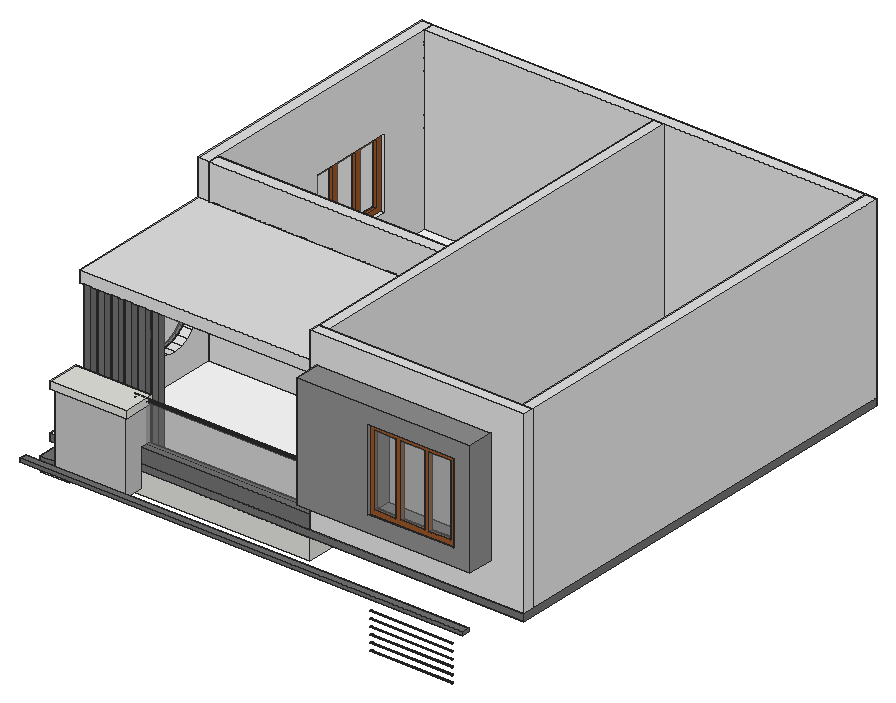
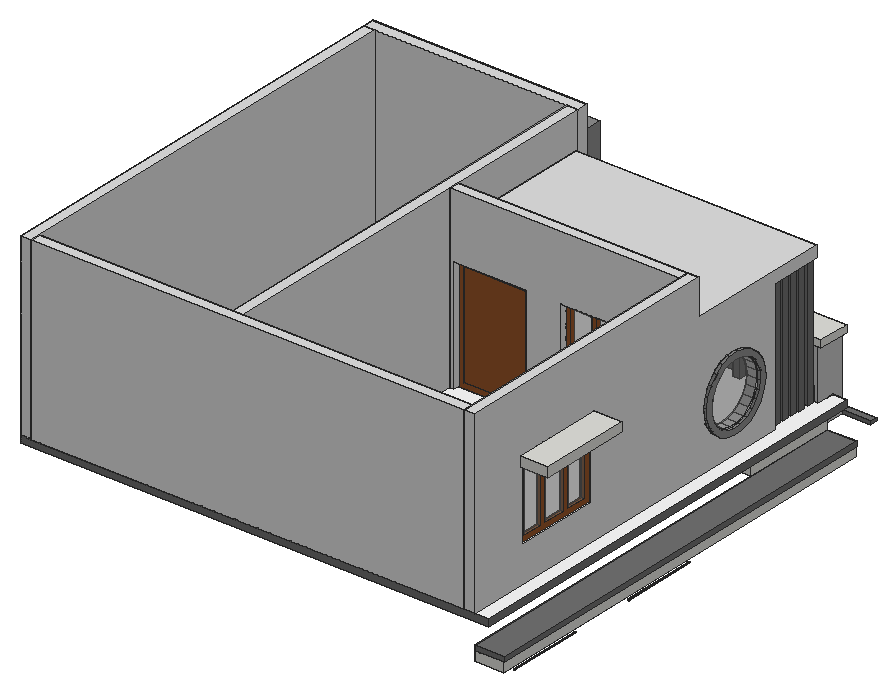
# SketchUp Ruby script. Lengths in inches.
U = 1.inch
M = Sketchup.active_model
def pt(a) = Geom::Point3d.new(a.map { |v| v * U })
def face(e, loops, mat)
  f = e.add_face(loops[0].map { |a| pt(a) })
  loops[1..].each { |l| e.add_face(l.map { |a| pt(a) }).erase! }
  f.material = f.back_material = mat if mat
  f
end
# faces: each face lists its corners as indices into pts; further lists are holes
def faces(e, pts, list, mat = nil) = list.each { |f| face(e, (f[0].is_a?(Array) ? f : [f]).map { |l| l.map { |i| pts[i] } }, mat) }
# xy, xz, yz: faces in a plane at the given z, y or x. An outline is a flat list of corners, or four numbers for a rectangle; further outlines are holes
def ring(l) = l.size == 4 ? [[l[0], l[1]], [l[2], l[1]], [l[2], l[3]], [l[0], l[3]]] : l.each_slice(2).to_a
def flat(e, list, mat, &to3) = list.each { |f| face(e, (f[0].is_a?(Array) ? f : [f]).map { |l| ring(l).map { |u, v| to3.(u, v) } }, mat) }
def xy(e, z, list, mat = nil) = flat(e, list, mat) { |x, y| [x, y, z] }
def xz(e, y, list, mat = nil) = flat(e, list, mat) { |x, z| [x, y, z] }
def yz(e, x, list, mat = nil) = flat(e, list, mat) { |y, z| [x, y, z] }
def lines(e, pts, list) = list.each { |a, b| e.add_line(pt(pts[a]), pt(pts[b])) }
# prism: a flat outline (further loops are holes) pulled along v
def prism(e, loops, v, mat = nil)
  f = face(e, loops, mat); d = Geom::Vector3d.new(v.map { |x| x * U })
  f.pushpull(f.normal.samedirection?(d) ? d.length : -d.length)
end
def box(e, o, s, mat = nil) = prism(e, [[o, [o[0] + s[0], o[1], o[2]], [o[0] + s[0], o[1] + s[1], o[2]], [o[0], o[1] + s[1], o[2]]]], [0, 0, s[2]], mat)
def at(x, y, z, deg = 0) = Geom::Transformation.translation(pt([x, y, z])) * Geom::Transformation.rotation(ORIGIN, Z_AXIS, deg.degrees)
def axes(o, x, y, z) = Geom::Transformation.new([*x, 0, *y, 0, *z, 0, *pt(o).to_a, 1])
def part(name) = M.definitions.add(name)
# library, detail: a bought-in or finely detailed component or shape, given as its bounding box
def library(name, o, s) = part(name).tap { |d| box(d.entities, o, s) }
def detail(e, o, s) = box(e.add_group.entities, o, s)
def put(e, d, t, mat = nil) = e.add_instance(d, t).tap { |i| i.material = mat if mat }
def group(e, t, mat = nil) = e.add_group.tap { |g| g.transformation = t; g.material = mat if mat }.entities
root = M.entities
M.materials.add("[Color M00]").color = [255, 255, 255]
M.materials.add("[Color M01]").color = [226, 226, 226]
M.materials.add("[Color M02]").color = [198, 198, 198]
M.materials.add("[Color M04]").color = [142, 142, 142]
M.materials.add("[Color M05]").color = [114, 114, 114]
M.materials.add("[Metal Silver]").color = [234, 233, 238]
M.materials.add("[Translucent Glass Gray]").color = [128, 128, 128]
M.materials["[Translucent Glass Gray]"].alpha = 0.5
M.materials.add("[Wood Cherry Original]").color = [152, 86, 42]
c1 = part("Group\#25")
prism(c1.entities,[[[0.28,64,0.08],[0.16,64,0.16],[0.08,64,0.28],[0.02,64,0.42],[0,64,0.5625],[0.02,64,0.71],[0.08,64,0.84],[0.16,64,0.96],[0.28,64,1.05],[0.42,64,1.11],[0.5625,64,1.125],[0.71,64,1.11],[0.84,64,1.05],[0.96,64,0.96],[1.05,64,0.84],[1.11,64,0.71],[1.125,64,0.5625],[1.11,64,0.42],[1.05,64,0.28],[0.96,64,0.16],[0.84,64,0.08],[0.71,64,0.02],[0.5625,64,0],[0.42,64,0.02]]],[0,-64,0])
c2 = part("Group\#30")
prism(c2.entities,[[[0.15,64,0.15],[0.07,64,0.25],[0.02,64,0.37],[0,64,0.5],[0.02,64,0.63],[0.07,64,0.75],[0.15,64,0.85],[0.25,64,0.93],[0.37,64,0.98],[0.5,64,1],[0.63,64,0.98],[0.75,64,0.93],[0.85,64,0.85],[0.93,64,0.75],[0.98,64,0.63],[1,64,0.5],[0.98,64,0.37],[0.93,64,0.25],[0.85,64,0.15],[0.75,64,0.07],[0.63,64,0.02],[0.5,64,0],[0.37,64,0.02],[0.25,64,0.07]]],[0,-64,0])
c3 = part("Group\#18")
prism(c3.entities,[[[0,1.11,0.71],[0,1.125,0.5625],[0,1.11,0.42],[0,1.05,0.28],[0,0.96,0.16],[0,0.84,0.08],[0,0.71,0.02],[0,0.5625,0],[0,0.42,0.02],[0,0.28,0.08],[0,0.16,0.16],[0,0.08,0.28],[0,0.02,0.42],[0,0,0.5625],[0,0.02,0.71],[0,0.08,0.84],[0,0.16,0.96],[0,0.28,1.05],[0,0.42,1.11],[0,0.5625,1.125],[0,0.71,1.11],[0,0.84,1.05],[0,0.96,0.96],[0,1.05,0.84]]],[64,0,0])
c4 = part("Group\#73")
box(c4.entities,[0,0,0],[6,4.96,110])
g1 = group(root,at(352.33,147.5,84.5))
prism(g1,[[[64,0.11,0.64],[64,0.05,0.5625],[64,0.01,0.47],[64,0,0.375],[64,0.01,0.28],[64,0.05,0.1875],[64,0.11,0.11],[64,0.1875,0.05],[64,0.28,0.01],[64,0.375,0],[64,0.47,0.01],[64,0.5625,0.05],[64,0.64,0.11],[64,0.7,0.1875],[64,0.74,0.28],[64,0.75,0.375],[64,0.74,0.47],[64,0.7,0.5625],[64,0.64,0.64],[64,0.5625,0.7],[64,0.47,0.74],[64,0.375,0.75],[64,0.28,0.74],[64,0.1875,0.7]]],[-69,0,0])
put(root,c1,at(87.27,300.375,86.45))
put(root,c2,at(87.33,420.375,86.78))
put(root,c3,at(137.33,242.3125,89.07))
g2 = group(root,at(352.33,147.5,90.5))
prism(g2,[[[64,0.11,0.64],[64,0.05,0.5625],[64,0.01,0.47],[64,0,0.375],[64,0.01,0.28],[64,0.05,0.1875],[64,0.11,0.11],[64,0.1875,0.05],[64,0.28,0.01],[64,0.375,0],[64,0.47,0.01],[64,0.5625,0.05],[64,0.64,0.11],[64,0.7,0.1875],[64,0.74,0.28],[64,0.75,0.375],[64,0.74,0.47],[64,0.7,0.5625],[64,0.64,0.64],[64,0.5625,0.7],[64,0.47,0.74],[64,0.375,0.75],[64,0.28,0.74],[64,0.1875,0.7]]],[-69,0,0])
put(root,c1,at(87.27,300.375,92.45))
put(root,c2,at(87.33,420.375,92.78))
put(root,c3,at(137.33,242.3125,95.07))
g3 = group(root,at(352.33,147.5,96.5))
prism(g3,[[[64,0.11,0.64],[64,0.05,0.5625],[64,0.01,0.47],[64,0,0.375],[64,0.01,0.28],[64,0.05,0.1875],[64,0.11,0.11],[64,0.1875,0.05],[64,0.28,0.01],[64,0.375,0],[64,0.47,0.01],[64,0.5625,0.05],[64,0.64,0.11],[64,0.7,0.1875],[64,0.74,0.28],[64,0.75,0.375],[64,0.74,0.47],[64,0.7,0.5625],[64,0.64,0.64],[64,0.5625,0.7],[64,0.47,0.74],[64,0.375,0.75],[64,0.28,0.74],[64,0.1875,0.7]]],[-69,0,0])
put(root,c1,at(87.27,300.375,98.45))
put(root,c2,at(87.33,420.375,98.78))
put(root,c3,at(137.33,242.3125,101.07))
g4 = group(root,at(352.33,147.5,102.5))
prism(g4,[[[64,0.11,0.64],[64,0.05,0.5625],[64,0.01,0.47],[64,0,0.375],[64,0.01,0.28],[64,0.05,0.1875],[64,0.11,0.11],[64,0.1875,0.05],[64,0.28,0.01],[64,0.375,0],[64,0.47,0.01],[64,0.5625,0.05],[64,0.64,0.11],[64,0.7,0.1875],[64,0.74,0.28],[64,0.75,0.375],[64,0.74,0.47],[64,0.7,0.5625],[64,0.64,0.64],[64,0.5625,0.7],[64,0.47,0.74],[64,0.375,0.75],[64,0.28,0.74],[64,0.1875,0.7]]],[-69,0,0])
put(root,c1,at(87.27,300.375,104.45))
put(root,c2,at(87.33,420.375,104.78))
put(root,c3,at(137.33,242.3125,107.07))
g5 = group(root,at(352.33,147.5,108.5))
prism(g5,[[[64,0.11,0.64],[64,0.05,0.5625],[64,0.01,0.47],[64,0,0.375],[64,0.01,0.28],[64,0.05,0.1875],[64,0.11,0.11],[64,0.1875,0.05],[64,0.28,0.01],[64,0.375,0],[64,0.47,0.01],[64,0.5625,0.05],[64,0.64,0.11],[64,0.7,0.1875],[64,0.74,0.28],[64,0.75,0.375],[64,0.74,0.47],[64,0.7,0.5625],[64,0.64,0.64],[64,0.5625,0.7],[64,0.47,0.74],[64,0.375,0.75],[64,0.28,0.74],[64,0.1875,0.7]]],[-69,0,0])
g6 = group(root,at(61.33,239.375,114))
box(g6,[0,-80,0],[24,369.8125,8])
g7 = group(root,at(352.33,147.5,114.5))
prism(g7,[[[64,0.11,0.64],[64,0.05,0.5625],[64,0.01,0.47],[64,0,0.375],[64,0.01,0.28],[64,0.05,0.1875],[64,0.11,0.11],[64,0.1875,0.05],[64,0.28,0.01],[64,0.375,0],[64,0.47,0.01],[64,0.5625,0.05],[64,0.64,0.11],[64,0.7,0.1875],[64,0.74,0.28],[64,0.75,0.375],[64,0.74,0.47],[64,0.7,0.5625],[64,0.64,0.64],[64,0.5625,0.7],[64,0.47,0.74],[64,0.375,0.75],[64,0.28,0.74],[64,0.1875,0.7]]],[-69,0,0])
g8 = group(root,at(60.33,239.375,122),"[Color M05]")
box(g8,[0,-80,0],[25,369.8125,4])
g9 = group(root,at(61.33,167.375,126))
box(g9,[24,-8,0],[202,80,18])
g10 = group(root,at(61.33,137.375,131),"[Color M05]")
box(g10,[0,0,0],[372,6,3])
g11 = group(root,at(85.33,143.375,131),"[Color M02]")
xy(g11,0,[[0,0,60,16]])
xy(g11,19,[[0,16,4,25]])
xy(g11,31,[[4,16,60,25]])
xy(g11,61,[[0,0,60,25]])
xz(g11,0,[[0,0,60,61]])
xz(g11,16,[[0,0,0,19,4,19,4,31,60,31,60,0]])
xz(g11,25,[[0,19,0,61,60,61,60,31,4,31,4,19]])
yz(g11,0,[[0,0,0,61,25,61,25,19,16,19,16,0]])
yz(g11,4,[[16,19,25,31]])
yz(g11,60,[[0,0,16,0,16,31,25,31,25,61,0,61]])
g12 = group(root,at(85.33,239.375,144),"[Color M05]")
xy(g12,0,[[-12,-86,-12,289.8125,382,289.8125,382,-80,0,-80,0,-86]])
xy(g12,6,[[-12,-86,0,-86,0,-80,382,-80,382,289.8125,-12,289.8125]],"[Color M00]")
xz(g12,-86,[[-12,0,0,6]])
xz(g12,-80,[[0,0,382,6]])
xz(g12,289.8125,[[-12,0,382,6]])
yz(g12,-12,[[-86,0,289.8125,6]])
yz(g12,0,[[-86,0,-80,6]])
yz(g12,382,[[-80,0,289.8125,6]])
g13 = group(root,at(287.33,159.375,150),"[Color M01]")
box(g13,[0,0,0],[180,9,150])
g14 = group(root,at(287.33,168.375,150),"[Color M01]")
box(g14,[0,0,0],[9,351.8125,150])
g15 = group(root,at(458.33,168.375,150),"[Color M01]")
box(g15,[0,0,0],[9,360.8125,150])
g16 = group(root,at(76.33,294.375,150),"[Color M01]")
prism(g16,[[[211,9,0],[207,9,0],[207,9,96],[147,9,96],[147,9,0],[18,9,0],[18,9,150],[211,9,150]],[[117,9,96],[45,9,96],[45,9,30],[117,9,30]]],[0,-9,0])
g17 = group(root,at(85.33,255.375,150),"[Color M01]")
xy(g17,0,[[0,-41,9,273.8125]])
xy(g17,30,[[0,152,9,224]])
xy(g17,90,[[0,152,9,224]])
xy(g17,110,[[0,-85,0,-41,9,-41,9,39,202,39,202,-85]])
xy(g17,120,[[0,-85,202,39]])
xy(g17,150,[[0,39,9,273.8125]])
xz(g17,-85,[[0,110,202,120]])
xz(g17,-41,[[0,0,9,110]])
xz(g17,39,[[9,110,202,120],[0,120,9,150]])
xz(g17,152,[[0,30,9,90]])
xz(g17,224,[[0,30,9,90]])
xz(g17,273.8125,[[0,0,9,150]])
yz(g17,-3,[[[4.67,17.04,-3.4,17.67,-11.03,20.36,-17.71,24.93,-22.97,31.08,-26.47,38.38,-27.96,46.33,-27.33,54.4,-24.64,62.03,-20.07,68.71,-13.92,73.97,-6.62,77.47,1.33,78.96,9.4,78.33,17.03,75.64,23.71,71.07,28.97,64.92,32.47,57.62,33.96,49.67,33.33,41.6,30.64,33.97,26.07,27.29,19.92,22.03,12.62,18.53],[4.4,22.04,11.07,23.28,17.19,26.22,22.35,30.63,26.18,36.23,28.44,42.63,28.96,49.4,27.72,56.07,24.78,62.19,20.37,67.35,14.77,71.18,8.37,73.44,1.6,73.96,-5.07,72.72,-11.19,69.78,-16.35,65.37,-20.18,59.77,-22.44,53.37,-22.96,46.6,-21.72,39.93,-18.78,33.81,-14.37,28.65,-8.77,24.82,-2.37,22.56]]],"[Color M04]")
yz(g17,0,[[[-41,0,-41,110,-85,110,-85,120,39,120,39,150,273.8125,150,273.8125,0],[152,30,224,90],[4.67,17.04,12.62,18.53,19.92,22.03,26.07,27.29,30.64,33.97,33.33,41.6,33.96,49.67,32.47,57.62,28.97,64.92,23.71,71.07,17.03,75.64,9.4,78.33,1.33,78.96,-6.62,77.47,-13.92,73.97,-20.07,68.71,-24.64,62.03,-27.33,54.4,-27.96,46.33,-26.47,38.38,-22.97,31.08,-17.71,24.93,-11.03,20.36,-3.4,17.67]],[[4.67,17.04,-3.4,17.67,-11.03,20.36,-17.71,24.93,-22.97,31.08,-26.47,38.38,-27.96,46.33,-27.33,54.4,-24.64,62.03,-20.07,68.71,-13.92,73.97,-6.62,77.47,1.33,78.96,9.4,78.33,17.03,75.64,23.71,71.07,28.97,64.92,32.47,57.62,33.96,49.67,33.33,41.6,30.64,33.97,26.07,27.29,19.92,22.03,12.62,18.53],[4.4,22.04,11.07,23.28,17.19,26.22,22.35,30.63,26.18,36.23,28.44,42.63,28.96,49.4,27.72,56.07,24.78,62.19,20.37,67.35,14.77,71.18,8.37,73.44,1.6,73.96,-5.07,72.72,-11.19,69.78,-16.35,65.37,-20.18,59.77,-22.44,53.37,-22.96,46.6,-21.72,39.93,-18.78,33.81,-14.37,28.65,-8.77,24.82,-2.37,22.56]]])
yz(g17,0,[[4.39,22.18,11.03,23.42,17.12,26.33,22.24,30.73,26.06,36.29,28.3,42.66,28.82,49.39,27.58,56.03,24.67,62.12,20.27,67.24,14.71,71.06,8.34,73.3,1.61,73.82,-5.03,72.58,-11.12,69.67,-16.24,65.27,-20.06,59.71,-22.3,53.34,-22.82,46.61,-21.58,39.97,-18.67,33.88,-14.27,28.76,-8.71,24.94,-2.34,22.7]],"[Translucent Glass Gray]")
yz(g17,9,[[[-41,0,273.8125,0,273.8125,150,39,150,39,110,-41,110],[152,30,224,90],[4.4,22.04,-2.37,22.56,-8.77,24.82,-14.37,28.65,-18.78,33.81,-21.72,39.93,-22.96,46.6,-22.44,53.37,-20.18,59.77,-16.35,65.37,-11.19,69.78,-5.07,72.72,1.6,73.96,8.37,73.44,14.77,71.18,20.37,67.35,24.78,62.19,27.72,56.07,28.96,49.4,28.44,42.63,26.18,36.23,22.35,30.63,17.19,26.22,11.07,23.28]]])
yz(g17,202,[[-85,110,39,120]])
p = [[0,4.67,17.04],[0,-3.4,17.67],[-3,-3.4,17.67],[-3,4.67,17.04],[0,12.62,18.53],[-3,12.62,18.53],
  [0,-11.03,20.36],[-3,-11.03,20.36],[0,19.92,22.03],[-3,19.92,22.03],[0,-17.71,24.93],[-3,-17.71,24.93],
  [0,-2.37,22.56],[0,4.4,22.04],[-3,4.4,22.04],[-3,-2.37,22.56],[9,-2.37,22.56],[9,4.4,22.04],
  [0,11.07,23.28],[-3,11.07,23.28],[9,11.07,23.28],[0,26.07,27.29],[-3,26.07,27.29],[0,-8.77,24.82],
  [-3,-8.77,24.82],[9,-8.77,24.82],[0,17.19,26.22],[-3,17.19,26.22],[9,17.19,26.22],[0,-14.37,28.65],
  [-3,-14.37,28.65],[9,-14.37,28.65],[0,-22.97,31.08],[-3,-22.97,31.08],[0,22.35,30.63],[-3,22.35,30.63],
  [9,22.35,30.63],[0,30.64,33.97],[-3,30.64,33.97],[0,-18.78,33.81],[-3,-18.78,33.81],[9,-18.78,33.81],
  [0,26.18,36.23],[-3,26.18,36.23],[9,26.18,36.23],[0,-26.47,38.38],[-3,-26.47,38.38],[0,-21.72,39.93],
  [-3,-21.72,39.93],[9,-21.72,39.93],[0,33.33,41.6],[-3,33.33,41.6],[0,28.44,42.63],[-3,28.44,42.63],
  [9,28.44,42.63],[0,-27.96,46.33],[-3,-27.96,46.33],[0,-22.96,46.6],[-3,-22.96,46.6],[9,-22.96,46.6],
  [0,33.96,49.67],[-3,33.96,49.67],[0,28.96,49.4],[-3,28.96,49.4],[9,28.96,49.4],[0,-27.33,54.4],
  [-3,-27.33,54.4],[0,-22.44,53.37],[-3,-22.44,53.37],[9,-22.44,53.37],[0,27.72,56.07],[-3,27.72,56.07],
  [9,27.72,56.07],[0,32.47,57.62],[-3,32.47,57.62],[0,-20.18,59.77],[-3,-20.18,59.77],[9,-20.18,59.77],
  [0,-24.64,62.03],[-3,-24.64,62.03],[0,24.78,62.19],[-3,24.78,62.19],[9,24.78,62.19],[0,28.97,64.92],
  [-3,28.97,64.92],[0,-16.35,65.37],[-3,-16.35,65.37],[9,-16.35,65.37],[0,-20.07,68.71],[-3,-20.07,68.71],
  [0,20.37,67.35],[-3,20.37,67.35],[9,20.37,67.35],[0,23.71,71.07],[-3,23.71,71.07],[0,-11.19,69.78],
  [-3,-11.19,69.78],[9,-11.19,69.78],[0,14.77,71.18],[-3,14.77,71.18],[9,14.77,71.18],[0,-13.92,73.97],
  [-3,-13.92,73.97],[0,-5.07,72.72],[-3,-5.07,72.72],[9,-5.07,72.72],[0,17.03,75.64],[-3,17.03,75.64],
  [0,8.37,73.44],[-3,8.37,73.44],[9,8.37,73.44],[0,1.6,73.96],[-3,1.6,73.96],[9,1.6,73.96],
  [0,-6.62,77.47],[-3,-6.62,77.47],[0,9.4,78.33],[-3,9.4,78.33],[0,1.33,78.96],[-3,1.33,78.96]]
faces(g17,p,[[0,1,2,3],[4,0,3,5],[1,6,7,2],[8,4,5,9],[6,10,11,7],[12,13,14,15],[13,18,19,14],[21,8,9,22],
  [23,12,15,24],[18,26,27,19],[29,23,24,30],[10,32,33,11],[26,34,35,27],[37,21,22,38],[39,29,30,40],[34,42,43,35],
  [32,45,46,33],[47,39,40,48],[50,37,38,51],[42,52,53,43],[45,55,56,46],[57,47,48,58],[60,50,51,61],[52,62,63,53],
  [55,65,66,56],[67,57,58,68],[62,70,71,63],[73,60,61,74],[75,67,68,76],[65,78,79,66],[70,80,81,71],[83,73,74,84],
  [85,75,76,86],[78,88,89,79],[80,90,91,81],[93,83,84,94],[95,85,86,96],[90,98,99,91],[88,101,102,89],[103,95,96,104],
  [106,93,94,107],[98,108,109,99],[111,103,104,112],[108,111,112,109],[101,114,115,102],[116,106,107,117],[114,118,119,115],[118,116,117,119]],"[Color M04]")
faces(g17,p,[[13,12,16,17],[18,13,17,20],[12,23,25,16],[26,18,20,28],[23,29,31,25],[34,26,28,36],[29,39,41,31],[42,34,36,44],
  [39,47,49,41],[52,42,44,54],[47,57,59,49],[62,52,54,64],[57,67,69,59],[70,62,64,72],[67,75,77,69],[80,70,72,82],
  [75,85,87,77],[90,80,82,92],[85,95,97,87],[98,90,92,100],[95,103,105,97],[108,98,100,110],[103,111,113,105],[111,108,110,113]])
g18 = group(root,at(85.33,159.375,150),"[Color M05]")
box(g18,[4,0,0],[198,9,12])
g19 = group(root,at(85.33,520.1875,150),"[Color M01]")
box(g19,[9,0,0],[364,9,150])
g20 = group(root,at(223.33,294.375,150),"[Wood Cherry Original]")
prism(g20,[[[60,4,0],[0,4,0],[0,4,96],[60,4,96]],[[4,4,4],[56,4,4],[56,4,92],[4,4,92]]],[0,-4,0])
put(root,c4,at(88.33,204.8,150),"[Color M05]")
put(root,c4,at(88.33,196.61,150),"[Color M05]")
put(root,c4,at(88.33,188.42,150),"[Color M05]")
put(root,c4,at(88.33,180.24,150),"[Color M05]")
put(root,c4,at(100.33,170.24,150),"[Color M05]")
put(root,c4,at(111.6,170.24,150),"[Color M05]")
put(root,c4,at(122.86,170.24,150),"[Color M05]")
put(root,c4,at(134.13,170.24,150),"[Color M05]")
put(root,c4,at(145.39,170.24,150),"[Color M05]")
put(root,c4,at(88.33,170.24,150),"[Color M05]")
g21 = group(root,at(227.33,296.375,154),"[Wood Cherry Original]")
xy(g21,0,[[5.75,-1,5.75,0,0,0,0,2,52,2,52,0,11.47,0,11.47,-1,10.71,-1,10.71,0,6.58,0,6.58,-1]])
xy(g21,8.72,[[24,-1,45.69,0]])
xy(g21,9.72,[[25,-1,44.69,0]])
xy(g21,14.1,[[29.39,0,40.31,0.3]])
xy(g21,15.1,[[30.39,-1,39.31,0.3]])
xy(g21,26.15,[[30.39,-1,39.31,0.3]])
xy(g21,27.15,[[29.39,0,40.31,0.3]])
xy(g21,31.53,[[25,-1,44.69,0]])
xy(g21,32.53,[[24,-1,45.69,0]])
xy(g21,44.86,[[24,-1,44.69,0]])
xy(g21,45.86,[[25,-1,43.69,0]])
xy(g21,51.24,[[30.375,0,38.32,0.3]])
xy(g21,52.24,[[31.375,-1,37.32,0.3]])
xy(g21,73.68,[[31.375,-1,37.32,0.3]])
xy(g21,74.68,[[30.375,0,38.32,0.3]])
xy(g21,80.05,[[25,-1,43.69,0]])
xy(g21,81.05,[[24,-1,44.69,0]])
xy(g21,88,[[5.75,-1,6.58,-1,6.58,0,10.71,0,10.71,-1,11.47,-1,11.47,0,52,0,52,2,0,2,0,0,5.75,0]])
xz(g21,-1,[[5.75,0,6.58,88],[10.71,0,11.47,88],[[24,8.72,45.69,32.53],[25,9.72,44.69,31.53]],[30.39,15.1,39.31,26.15],[[24,44.86,44.69,81.05],[25,45.86,43.69,80.05]],
  [31.375,52.24,37.32,73.68]])
xz(g21,0,[[0,0,5.75,88],[6.58,0,10.71,88],[[11.47,0,52,88],[24,44.86,44.69,81.05],[24,8.72,45.69,32.53]],[[25,9.72,44.69,31.53],[29.39,14.1,40.31,27.15]],[[25,45.86,43.69,80.05],[30.375,51.24,38.32,74.68]]])
xz(g21,0.3,[[[29.39,14.1,40.31,27.15],[30.39,15.1,39.31,26.15]],[[30.375,51.24,38.32,74.68],[31.375,52.24,37.32,73.68]]])
xz(g21,2,[[0,0,52,88]])
yz(g21,0,[[0,0,2,88]])
yz(g21,5.75,[[-1,0,0,88]])
yz(g21,6.58,[[-1,0,0,88]])
yz(g21,10.71,[[-1,0,0,88]])
yz(g21,11.47,[[-1,0,0,88]])
yz(g21,24,[[-1,8.72,0,32.53],[-1,44.86,0,81.05]])
yz(g21,25,[[-1,9.72,0,31.53],[-1,45.86,0,80.05]])
yz(g21,29.39,[[0,14.1,0.3,27.15]])
yz(g21,30.375,[[0,51.24,0.3,74.68]])
yz(g21,30.39,[[-1,15.1,0.3,26.15]])
yz(g21,31.375,[[-1,52.24,0.3,73.68]])
yz(g21,37.32,[[-1,52.24,0.3,73.68]])
yz(g21,38.32,[[0,51.24,0.3,74.68]])
yz(g21,39.31,[[-1,15.1,0.3,26.15]])
yz(g21,40.31,[[0,14.1,0.3,27.15]])
yz(g21,43.69,[[-1,45.86,0,80.05]])
yz(g21,44.69,[[-1,9.72,0,31.53],[-1,44.86,0,81.05]])
yz(g21,45.69,[[-1,8.72,0,32.53]])
yz(g21,52,[[0,0,2,88]])
g22 = group(root,at(135.33,164.625,162),"[Translucent Glass Gray]")
xz(g22,0,[[0,0,152,33.84]])
g23 = group(root,at(293.33,137.375,180),"[Color M04]")
prism(g23,[[[0,0,96],[0,0,0],[146,0,0],[146,0,96]],[[60,0,14],[60,0,82],[132,0,82],[132,0,14]]],[0,22,0])
g24 = group(root,at(87.33,407.375,180),"[Wood Cherry Original]")
prism(g24,[[[0,0,60],[0,72,60],[0,72,0],[0,0,0]],[[0,26,4],[0,46,4],[0,46,56],[0,26,56]],[[0,22,4],[0,22,56],[0,4,56],[0,4,4]],[[0,50,56],[0,50,4],[0,68,4],[0,68,56]]],[3,0,0])
g25 = group(root,at(121.33,295.375,180),"[Wood Cherry Original]")
prism(g25,[[[0,3,66],[72,3,66],[72,3,0],[0,3,0]],[[26,3,4],[46,3,4],[46,3,62],[26,3,62]],[[22,3,4],[22,3,62],[4,3,62],[4,3,4]],[[50,3,62],[50,3,4],[68,3,4],[68,3,62]]],[0,-3,0])
g26 = group(root,at(228.84,294.375,180.41),"[Metal Silver]")
prism(g26,[[[2.0625,2,24.7],[2.0625,2,26.4375],[2.0625,0,26.4375],[2.0625,0,0],[2.0625,2,0],[2.0625,2,1.73],[2.0625,0.73,1.73],[2.0625,0.73,24.7]]],[-2.0625,0,0])
g27 = group(root,at(87.33,411.375,184),"[Translucent Glass Gray]")
yz(g27,0,[[0,0,18,52]])
g28 = group(root,at(87.33,433.375,184),"[Translucent Glass Gray]")
yz(g28,0,[[0,0,20,52]])
g29 = group(root,at(87.33,457.375,184),"[Translucent Glass Gray]")
yz(g29,0,[[0,0,18,52]])
g30 = group(root,at(171.33,295.375,184),"[Translucent Glass Gray]")
xz(g30,0,[[0,0,18,58]])
g31 = group(root,at(147.33,295.375,184),"[Translucent Glass Gray]")
xz(g31,0,[[0,0,20,58]])
g32 = group(root,at(125.33,295.375,184),"[Translucent Glass Gray]")
xz(g32,0,[[0,0,18,58]])
g33 = group(root,at(83.33,141.375,192))
box(g33,[0,0,0],[64,27,6])
g34 = group(root,at(353.33,139.375,194),"[Wood Cherry Original]")
prism(g34,[[[0,3,68],[72,3,68],[72,3,0],[0,3,0]],[[26,3,4],[46,3,4],[46,3,64],[26,3,64]],[[22,3,4],[22,3,64],[4,3,64],[4,3,4]],[[50,3,64],[50,3,4],[68,3,4],[68,3,64]]],[0,-3,0])
g35 = group(root,at(135.33,163.4375,194.32),"[Metal Silver]")
prism(g35,[[[0,1.78,2.22],[0,2.03,2.03],[0,2.22,1.78],[0,2.33,1.49],[0,2.375,1.1875],[0,2.33,0.88],[0,2.22,0.59],[0,2.03,0.35],[0,1.78,0.16],[0,1.49,0.04],[0,1.1875,0],[0,0.88,0.04],[0,0.59,0.16],[0,0.35,0.35],[0,0.16,0.59],[0,0.04,0.88],[0,0,1.1875],[0,0.04,1.49],[0,0.16,1.78],[0,0.35,2.03],[0,0.59,2.22],[0,0.88,2.33],[0,1.1875,2.375],[0,1.49,2.33]]],[158,0,0])
g36 = group(root,at(403.33,139.375,198),"[Translucent Glass Gray]")
xz(g36,0,[[0,0,18,60]])
g37 = group(root,at(379.33,139.375,198),"[Translucent Glass Gray]")
xz(g37,0,[[0,0,20,60]])
g38 = group(root,at(357.33,139.375,198),"[Translucent Glass Gray]")
xz(g38,0,[[0,0,18,60]])
g39 = group(root,at(61.33,404.375,240))
box(g39,[0,0,0],[24,78,8])
